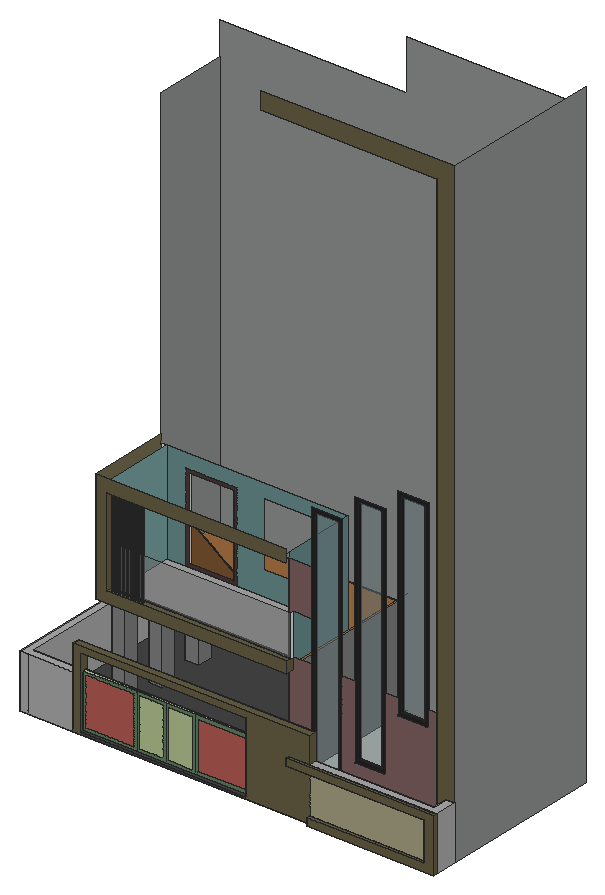
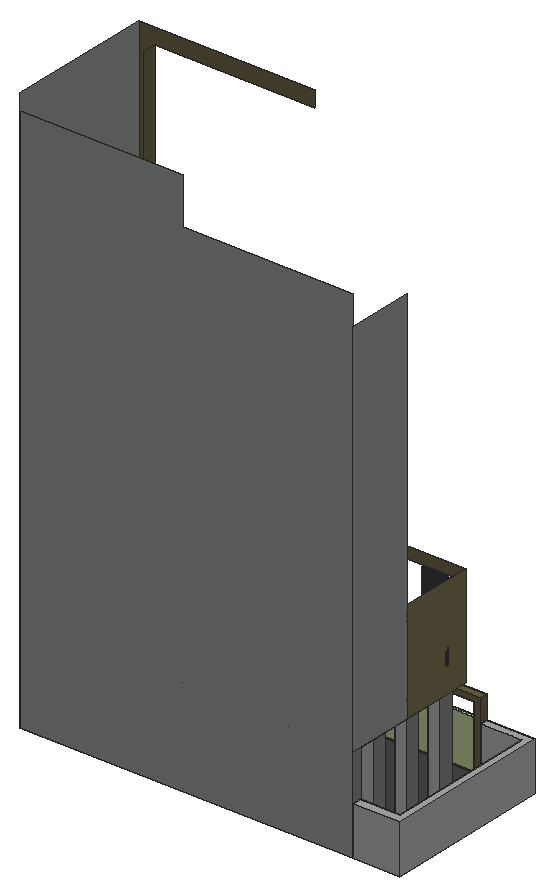
# SketchUp Ruby script. Lengths in inches.
U = 1.inch
M = Sketchup.active_model
def pt(a) = Geom::Point3d.new(a.map { |v| v * U })
def face(e, loops, mat)
  f = e.add_face(loops[0].map { |a| pt(a) })
  loops[1..].each { |l| e.add_face(l.map { |a| pt(a) }).erase! }
  f.material = f.back_material = mat if mat
  f
end
# faces: each face lists its corners as indices into pts; further lists are holes
def faces(e, pts, list, mat = nil) = list.each { |f| face(e, (f[0].is_a?(Array) ? f : [f]).map { |l| l.map { |i| pts[i] } }, mat) }
# xy, xz, yz: faces in a plane at the given z, y or x. An outline is a flat list of corners, or four numbers for a rectangle; further outlines are holes
def ring(l) = l.size == 4 ? [[l[0], l[1]], [l[2], l[1]], [l[2], l[3]], [l[0], l[3]]] : l.each_slice(2).to_a
def flat(e, list, mat, &to3) = list.each { |f| face(e, (f[0].is_a?(Array) ? f : [f]).map { |l| ring(l).map { |u, v| to3.(u, v) } }, mat) }
def xy(e, z, list, mat = nil) = flat(e, list, mat) { |x, y| [x, y, z] }
def xz(e, y, list, mat = nil) = flat(e, list, mat) { |x, z| [x, y, z] }
def yz(e, x, list, mat = nil) = flat(e, list, mat) { |y, z| [x, y, z] }
def lines(e, pts, list) = list.each { |a, b| e.add_line(pt(pts[a]), pt(pts[b])) }
# prism: a flat outline (further loops are holes) pulled along v
def prism(e, loops, v, mat = nil)
  f = face(e, loops, mat); d = Geom::Vector3d.new(v.map { |x| x * U })
  f.pushpull(f.normal.samedirection?(d) ? d.length : -d.length)
end
def box(e, o, s, mat = nil) = prism(e, [[o, [o[0] + s[0], o[1], o[2]], [o[0] + s[0], o[1] + s[1], o[2]], [o[0], o[1] + s[1], o[2]]]], [0, 0, s[2]], mat)
def at(x, y, z, deg = 0) = Geom::Transformation.translation(pt([x, y, z])) * Geom::Transformation.rotation(ORIGIN, Z_AXIS, deg.degrees)
def axes(o, x, y, z) = Geom::Transformation.new([*x, 0, *y, 0, *z, 0, *pt(o).to_a, 1])
def part(name) = M.definitions.add(name)
# library, detail: a bought-in or finely detailed component or shape, given as its bounding box
def library(name, o, s) = part(name).tap { |d| box(d.entities, o, s) }
def detail(e, o, s) = box(e.add_group.entities, o, s)
def put(e, d, t, mat = nil) = e.add_instance(d, t).tap { |i| i.material = mat if mat }
def group(e, t, mat = nil) = e.add_group.tap { |g| g.transformation = t; g.material = mat if mat }.entities
root = M.entities
M.materials.add("[0072_DarkSeaGreen]").color = [96, 127, 96]
M.materials.add("[0089_PaleTurquoise]").color = [103, 140, 140]
M.materials.add("[0089_PaleTurquoise]1").color = [120, 163, 163]
M.materials.add("[0089_PaleTurquoise]2").color = [93, 127, 127]
M.materials.add("[0119_RosyBrown]").color = [127, 96, 96]
M.materials.add("[0119_RosyBrown]1").color = [76, 58, 58]
M.materials.add("[0132_LightGray]").color = [127, 127, 127]
M.materials.add("[0132_LightGray]1").color = [169, 169, 169]
M.materials.add("[0136_Charcoal]").color = [35, 35, 35]
M.materials.add("[Beadboard]").color = [178, 193, 144]
M.materials.add("[Blacktop Old 02]").color = [143, 145, 145]
M.materials.add("[Cladding Siding Tan]").color = [178, 91, 82]
M.materials.add("[Granite Dark Gray]").color = [69, 68, 68]
M.materials.add("[Granite Dark Gray]1").color = [69, 68, 68]
M.materials.add("[Stone Coursed Rough]").color = [165, 160, 130]
M.materials.add("[Stone Vein Gray]").color = [166, 165, 165]
M.materials.add("[Translucent Glass Gray]").color = [130, 130, 130]
M.materials["[Translucent Glass Gray]"].alpha = 0.5
M.materials.add("[Translucent Glass Safety]").color = [119, 137, 142]
M.materials["[Translucent Glass Safety]"].alpha = 0.5
M.materials.add("[Wood Floor]").color = [124, 84, 49]
M.materials.add("[Wood Floor]1").color = [155, 105, 61]
M.materials.add("[Wood Lumber ButtJoined]").color = [102, 94, 69]
M.materials.add("[Wood Lumber ButtJoined]2").color = [117, 108, 80]
xy(root,0,[[0,18,240,894],[240,18,1963.2,198],[240,198,1963.2,894]])
xy(root,0,[[1363.2,0,1963.2,18]],"[Wood Lumber ButtJoined]")
xy(root,12,[[285,32.01,1065,46.01],[249,246,312,318],[249,462,312,534],[249,678,312,750]])
xy(root,12,[[285,18,1065,32.01],[[36,54,1921.2,54,1921.2,126,1879.2,126,1879.2,198,1122,198,1122,846,36,846],[249,462,312,534],[249,246,312,318],[249,678,312,750]]],"[Granite Dark Gray]")
xy(root,12,[[285,46.01,1065,54]],"[Granite Dark Gray]1")
xy(root,30,[[1248,198,1356,208]],"[0136_Charcoal]")
xy(root,36,[[1363.2,0,1915.2,18]],"[Wood Lumber ButtJoined]")
xy(root,220.8,[[1267.2,0,1915.2,18]],"[Wood Lumber ButtJoined]")
xy(root,222,[[1452,198,1560,208]],"[0136_Charcoal]")
xy(root,252,[[0,18,249,18,249,54,36,54,36,846,240,846,240,894,0,894],[1363.2,18,1963.2,18,1963.2,126,1921.2,126,1921.2,54,1363.2,54]],"[0132_LightGray]1")
xy(root,252,[[1267.2,0,1963.2,18]],"[Wood Lumber ButtJoined]")
xy(root,264,[[285,32.01,1065,46.01]],"[Beadboard]")
xy(root,342,[[285,18,1065,54]],"[Wood Lumber ButtJoined]")
xy(root,372,[[249,18,1363.2,54]],"[Wood Lumber ButtJoined]")
xy(root,492,[[[240,198,1122,846],[249,462,312,534],[249,678,312,750],[249,246,312,318]]],"[Wood Floor]1")
xy(root,492,[[240,162,1140.5,198]],"[Wood Lumber ButtJoined]")
xy(root,492.0625,[[1656,198,1764,208]],"[0136_Charcoal]")
xy(root,504,[[270,198,1122,546]],"[Stone Vein Gray]")
xy(root,519.6,[[375.6,546,584.4,551]])
xy(root,546,[[294,189.55,1140.5,198]],"[0089_PaleTurquoise]2")
xy(root,546,[[[294,162,1140.5,189.55],[326.5625,171.77,325.53,171.91,324.5625,172.31,323.73,172.94,323.1,173.77,322.7,174.74,322.5625,175.77,322.7,176.81,323.1,177.77,323.73,178.6,324.5625,179.24,325.53,179.64,326.5625,179.77,327.6,179.64,328.5625,179.24,329.39,178.6,330.03,177.77,330.43,176.81,330.5625,175.77,330.43,174.74,330.03,173.77,329.39,172.94,328.5625,172.31,327.6,171.91],[344.5625,171.77,343.53,171.91,342.5625,172.31,341.73,172.94,341.1,173.77,340.7,174.74,340.5625,175.77,340.7,176.81,341.1,177.77,341.73,178.6,342.5625,179.24,343.53,179.64,344.5625,179.77,345.6,179.64,346.5625,179.24,347.39,178.6,348.03,177.77,348.43,176.81,348.5625,175.77,348.43,174.74,348.03,173.77,347.39,172.94,346.5625,172.31,345.6,171.91],[362.5625,171.77,361.53,171.91,360.5625,172.31,359.73,172.94,359.1,173.77,358.7,174.74,358.5625,175.77,358.7,176.81,359.1,177.77,359.73,178.6,360.5625,179.24,361.53,179.64,362.5625,179.77,363.6,179.64,364.5625,179.24,365.39,178.6,366.03,177.77,366.43,176.81,366.5625,175.77,366.43,174.74,366.03,173.77,365.39,172.94,364.5625,172.31,363.6,171.91],[380.5625,171.77,379.53,171.91,378.5625,172.31,377.73,172.94,377.1,173.77,376.7,174.74,376.5625,175.77,376.7,176.81,377.1,177.77,377.73,178.6,378.5625,179.24,379.53,179.64,380.5625,179.77,381.6,179.64,382.5625,179.24,383.39,178.6,384.03,177.77,384.43,176.81,384.5625,175.77,384.43,174.74,384.03,173.77,383.39,172.94,382.5625,172.31,381.6,171.91],[398.5625,171.77,397.53,171.91,396.5625,172.31,395.73,172.94,395.1,173.77,394.7,174.74,394.5625,175.77,394.7,176.81,395.1,177.77,395.73,178.6,396.5625,179.24,397.53,179.64,398.5625,179.77,399.6,179.64,400.5625,179.24,401.39,178.6,402.03,177.77,402.43,176.81,402.5625,175.77,402.43,174.74,402.03,173.77,401.39,172.94,400.5625,172.31,399.6,171.91],[416.5625,171.77,415.53,171.91,414.5625,172.31,413.73,172.94,413.1,173.77,412.7,174.74,412.5625,175.77,412.7,176.81,413.1,177.77,413.73,178.6,414.5625,179.24,415.53,179.64,416.5625,179.77,417.6,179.64,418.5625,179.24,419.39,178.6,420.03,177.77,420.43,176.81,420.5625,175.77,420.43,174.74,420.03,173.77,419.39,172.94,418.5625,172.31,417.6,171.91],[434.5625,171.77,433.53,171.91,432.5625,172.31,431.73,172.94,431.1,173.77,430.7,174.74,430.5625,175.77,430.7,176.81,431.1,177.77,431.73,178.6,432.5625,179.24,433.53,179.64,434.5625,179.77,435.6,179.64,436.5625,179.24,437.39,178.6,438.03,177.77,438.43,176.81,438.5625,175.77,438.43,174.74,438.03,173.77,437.39,172.94,436.5625,172.31,435.6,171.91],[452.5625,171.77,451.53,171.91,450.5625,172.31,449.73,172.94,449.1,173.77,448.7,174.74,448.5625,175.77,448.7,176.81,449.1,177.77,449.73,178.6,450.5625,179.24,451.53,179.64,452.5625,179.77,453.6,179.64,454.5625,179.24,455.39,178.6,456.03,177.77,456.43,176.81,456.5625,175.77,456.43,174.74,456.03,173.77,455.39,172.94,454.5625,172.31,453.6,171.91],[308.5625,171.77,307.53,171.91,306.5625,172.31,305.73,172.94,305.1,173.77,304.7,174.74,304.5625,175.77,304.7,176.81,305.1,177.77,305.73,178.6,306.5625,179.24,307.53,179.64,308.5625,179.77,309.6,179.64,310.5625,179.24,311.39,178.6,312.03,177.77,312.43,176.81,312.5625,175.77,312.43,174.74,312.03,173.77,311.39,172.94,310.5625,172.31,309.6,171.91]]],"[Wood Lumber ButtJoined]")
xz(root,0,[[1363.2,0,1963.2,0,1963.2,252,1267.2,252,1267.2,220.8,1915.2,220.8,1915.2,36,1363.2,36]],"[Wood Lumber ButtJoined]")
xz(root,18,[[1363.2,0,1363.2,36,1915.2,36,1915.2,220.8,1267.2,220.8,1267.2,252,1963.2,252,1963.2,0]])
xz(root,18,[[0,0,36,252],[36,0,249,252]],"[0132_LightGray]1")
xz(root,18,[[285,0,1065,12]],"[Granite Dark Gray]")
xz(root,18,[[1363.2,36,1915.2,220.8]],"[Stone Coursed Rough]")
xz(root,18,[[249,0,285,0,285,342,1065,342,1065,0,1363.2,0,1363.2,220.8,1267.2,220.8,1267.2,252,1363.2,252,1363.2,372,249,372]],"[Wood Lumber ButtJoined]")
xz(root,32.01,[[[285,12,537,264],[299.4,26.4,522.6,249.6]],[[537,12,675,264],[551.4,26.4,660.6,249.6]],[[675,12,813,264],[689.4,26.4,798.6,249.6]],[[813,12,1065,264],[827.4,26.4,1050.6,249.6]]],"[0072_DarkSeaGreen]")
xz(root,32.01,[[551.4,26.4,660.6,249.6],[689.4,26.4,798.6,249.6]],"[Beadboard]")
xz(root,32.01,[[299.4,26.4,522.6,249.6],[827.4,26.4,1050.6,249.6]],"[Cladding Siding Tan]")
xz(root,46.01,[[285,12,1065,264]],"[Beadboard]")
xz(root,54,[[36,12,249,252],[1363.2,12,1921.2,252]],"[0132_LightGray]1")
xz(root,54,[[249,12,249,372,1363.2,372,1363.2,12,1065,12,1065,342,285,342,285,12]],"[Wood Lumber ButtJoined]")
xz(root,126,[[1921.2,12,1963.2,252]])
xz(root,126,[[1879.2,12,1921.2,12,1921.2,252,1963.2,252,1963.2,2940,1050,2940,1050,2856,1879.2,2856]],"[Wood Lumber ButtJoined]")
xz(root,162,[[240,492,1140.5,492,1140.5,546,294,546,294,960,1135.625,960,1135.625,1020,240,1020]],"[Wood Lumber ButtJoined]")
xz(root,189.55,[[294,546,1140.5,738]],"[Translucent Glass Gray]")
xz(root,198,[[1122,504,1140.5,546]])
xz(root,198,[[270,504,270,960,294,960,294,546,1122,546,1122,504]],"[0089_PaleTurquoise]2")
xz(root,198,[[1122,12,1230,12,1230,549.1875,1140.5,549.1875,1140.5,492,1122,492],[1374,12,1879.2,12,1879.2,549.1875,1782,549.1875,1782,474.0625,1638,474.0625,1638,549.1875,1578,549.1875,1578,204,1434,204,1434,549.1875,1374,549.1875],[1122,546,1140.5,546,1140.5,732,1138.98,732.2,1137.53,732.79,1136.28,733.73,1135.32,734.97,1134.71,736.42,1134.5,737.97,1134.7,739.52,1135.29,740.97,1136.23,742.22,1137.47,743.18,1138.92,743.79,1140.47,744,1142.02,743.8,1143.47,743.21,1144.72,742.27,1230,742.375,1230,958.375,1122,958.375]],"[0119_RosyBrown]")
xz(root,198,[[[1230,12,1374,1212],[1248,30,1356,1194]],[[1434,204,1578,1328.4375],[1452,222,1560,1310.4375]],[[1638,474.0625,1782,1424.375],[1656,492.0625,1764,1406.375]]],"[0136_Charcoal]")
xz(root,208,[[1248,30,1356,1194],[1452,222,1560,1310.4375],[1656,492.0625,1764,1406.375]],"[Translucent Glass Safety]")
xz(root,246,[[249,12,312,492]],"[0132_LightGray]")
xz(root,318,[[249,12,312,492]],"[0132_LightGray]1")
xz(root,462,[[249,12,312,492]],"[0132_LightGray]")
xz(root,534,[[249,12,312,492]],"[0132_LightGray]1")
xz(root,546,[[240,504,270,984]])
xz(root,546,[[[270,504,360,504,360,919.5,600,919.5,600,504,1122,504,1122,984,270,984],[726,619.5,973.25,919.5]]],"[0089_PaleTurquoise]")
xz(root,546,[[[360,504,600,919.5],[375.6,519.6,584.4,903.9]]],"[0119_RosyBrown]1")
xz(root,551,[[584.4,546.38,584.4,551.94,507.28,606.22,503.9375,608.57,379.5,696.14,375.6,692.98]])
xz(root,551,[[375.6,519.6,584.4,519.6,584.4,546.38,375.6,692.98]],"[Wood Floor]")
xz(root,678,[[249,12,312,492]],"[0132_LightGray]")
xz(root,750,[[249,12,312,492]],"[0132_LightGray]1")
xz(root,846,[[240,12,1122,492]],"[0132_LightGray]")
xz(root,846,[[36,12,240,252]],"[0132_LightGray]1")
xz(root,894,[[0,0,240,252]],"[0132_LightGray]1")
xz(root,894,[[240,0,240,2616,1122,2616,1122,2856,1963.2,2856,1963.2,0]],"[Blacktop Old 02]")
yz(root,0,[[18,0,894,252]],"[0132_LightGray]1")
yz(root,36,[[54,12,846,252]],"[0132_LightGray]1")
yz(root,240,[[846,12,894,252]])
yz(root,240,[[846,252,894,492]],"[0132_LightGray]")
yz(root,240,[[546,492,894,2460]],"[Blacktop Old 02]")
yz(root,240,[[162,492,546,1020]],"[Wood Lumber ButtJoined]2")
yz(root,249,[[18,12,54,252]])
yz(root,249,[[246,12,318,492],[462,12,534,492],[678,12,750,492]],"[0132_LightGray]")
yz(root,249,[[18,252,54,372]],"[Wood Lumber ButtJoined]")
yz(root,270,[[198,504,546,504,546,984,204,984,204,960,198,960]],"[0089_PaleTurquoise]1")
yz(root,285,[[32.01,12,46.01,264]])
yz(root,285,[[18,12,32.01,12,32.01,264,46.01,264,46.01,12,54,12,54,342,18,342]],"[Wood Lumber ButtJoined]")
yz(root,294,[[[162,546,198,960],[189.51,732,187.96,732.21,186.52,732.82,185.28,733.78,184.33,735.03,183.74,736.48,183.55,738.03,183.76,739.58,184.37,741.03,185.33,742.27,186.57,743.21,188.02,743.8,189.58,744,191.13,743.79,192.57,743.18,193.8125,742.22,194.76,740.97,195.35,739.52,195.55,737.97,195.33,736.42,194.72,734.97,193.76,733.73,192.52,732.79,191.07,732.2,189.55,732]]],"[Wood Lumber ButtJoined]")
yz(root,312,[[246,12,318,492],[462,12,534,492],[678,12,750,492]],"[0132_LightGray]")
yz(root,375.6,[[546,519.6,551,903.9]])
yz(root,584.4,[[546,519.6,551,903.9]])
yz(root,1065,[[32.01,12,46.01,264]])
yz(root,1065,[[18,12,18,342,54,342,54,12,46.01,12,46.01,264,32.01,264,32.01,12]],"[Wood Lumber ButtJoined]")
yz(root,1122,[[198,504,198,960,204,960,204,984,546,984,546,504]],"[0089_PaleTurquoise]")
yz(root,1122,[[198,12,846,492]],"[0132_LightGray]")
yz(root,1140.5,[[189.55,546,198,738]])
yz(root,1140.5,[[162,492,198,546]],"[Wood Lumber ButtJoined]")
yz(root,1248,[[198,30,208,1194]],"[0136_Charcoal]")
yz(root,1267.2,[[0,220.8,18,252]],"[Wood Lumber ButtJoined]")
yz(root,1356,[[198,30,208,1194]],"[0136_Charcoal]")
yz(root,1363.2,[[0,0,18,36],[18,252,54,372]],"[Wood Lumber ButtJoined]")
yz(root,1452,[[198,222,208,1310.4375]],"[0136_Charcoal]")
yz(root,1560,[[198,222,208,1310.4375]],"[0136_Charcoal]")
yz(root,1656,[[198,492.0625,208,1406.375]],"[0136_Charcoal]")
yz(root,1764,[[198,492.0625,208,1406.375]],"[0136_Charcoal]")
yz(root,1879.2,[[126,12,198,2856]],"[Wood Lumber ButtJoined]")
yz(root,1915.2,[[0,36,18,220.8]],"[Wood Lumber ButtJoined]")
yz(root,1921.2,[[54,12,126,252]],"[0132_LightGray]1")
yz(root,1963.2,[[18,0,126,252]],"[0132_LightGray]1")
yz(root,1963.2,[[126,0,894,2940]],"[Blacktop Old 02]")
yz(root,1963.2,[[0,0,18,252]],"[Wood Lumber ButtJoined]")
p = [[307.53,171.91,546],[308.5625,171.77,546],[308.5625,171.77,960],[307.53,171.91,960],[309.6,171.91,546],[309.6,171.91,960],
  [325.53,171.91,546],[326.5625,171.77,546],[326.5625,171.77,960],[325.53,171.91,960],[327.6,171.91,546],[327.6,171.91,960],
  [343.53,171.91,546],[344.5625,171.77,546],[344.5625,171.77,960],[343.53,171.91,960],[345.6,171.91,546],[345.6,171.91,960],
  [361.53,171.91,546],[362.5625,171.77,546],[362.5625,171.77,960],[361.53,171.91,960],[363.6,171.91,546],[363.6,171.91,960],
  [379.53,171.91,546],[380.5625,171.77,546],[380.5625,171.77,960],[379.53,171.91,960],[381.6,171.91,546],[381.6,171.91,960],
  [397.53,171.91,546],[398.5625,171.77,546],[398.5625,171.77,960],[397.53,171.91,960],[399.6,171.91,546],[399.6,171.91,960],
  [415.53,171.91,546],[416.5625,171.77,546],[416.5625,171.77,960],[415.53,171.91,960],[417.6,171.91,546],[417.6,171.91,960],
  [433.53,171.91,546],[434.5625,171.77,546],[434.5625,171.77,960],[433.53,171.91,960],[435.6,171.91,546],[435.6,171.91,960],
  [451.53,171.91,546],[452.5625,171.77,546],[452.5625,171.77,960],[451.53,171.91,960],[453.6,171.91,546],[453.6,171.91,960],
  [306.5625,172.31,546],[306.5625,172.31,960],[310.5625,172.31,546],[310.5625,172.31,960],[324.5625,172.31,546],[324.5625,172.31,960],
  [328.5625,172.31,546],[328.5625,172.31,960],[342.5625,172.31,546],[342.5625,172.31,960],[346.5625,172.31,546],[346.5625,172.31,960],
  [360.5625,172.31,546],[360.5625,172.31,960],[364.5625,172.31,546],[364.5625,172.31,960],[378.5625,172.31,546],[378.5625,172.31,960],
  [382.5625,172.31,546],[382.5625,172.31,960],[396.5625,172.31,546],[396.5625,172.31,960],[400.5625,172.31,546],[400.5625,172.31,960],
  [414.5625,172.31,546],[414.5625,172.31,960],[418.5625,172.31,546],[418.5625,172.31,960],[432.5625,172.31,546],[432.5625,172.31,960],
  [436.5625,172.31,546],[436.5625,172.31,960],[450.5625,172.31,546],[450.5625,172.31,960],[454.5625,172.31,546],[454.5625,172.31,960],
  [305.73,172.94,546],[305.73,172.94,960],[311.39,172.94,546],[311.39,172.94,960],[323.73,172.94,546],[323.73,172.94,960],
  [329.39,172.94,546],[329.39,172.94,960],[341.73,172.94,546],[341.73,172.94,960],[347.39,172.94,546],[347.39,172.94,960],
  [359.73,172.94,546],[359.73,172.94,960],[365.39,172.94,546],[365.39,172.94,960],[377.73,172.94,546],[377.73,172.94,960],
  [383.39,172.94,546],[383.39,172.94,960],[395.73,172.94,546],[395.73,172.94,960],[401.39,172.94,546],[401.39,172.94,960],
  [413.73,172.94,546],[413.73,172.94,960],[419.39,172.94,546],[419.39,172.94,960],[431.73,172.94,546],[431.73,172.94,960],
  [437.39,172.94,546],[437.39,172.94,960],[449.73,172.94,546],[449.73,172.94,960],[455.39,172.94,546],[455.39,172.94,960],
  [305.1,173.77,546],[305.1,173.77,960],[312.03,173.77,546],[312.03,173.77,960],[323.1,173.77,546],[323.1,173.77,960],
  [330.03,173.77,546],[330.03,173.77,960],[341.1,173.77,546],[341.1,173.77,960],[348.03,173.77,546],[348.03,173.77,960],
  [359.1,173.77,546],[359.1,173.77,960],[366.03,173.77,546],[366.03,173.77,960],[377.1,173.77,546],[377.1,173.77,960],
  [384.03,173.77,546],[384.03,173.77,960],[395.1,173.77,546],[395.1,173.77,960],[402.03,173.77,546],[402.03,173.77,960],
  [413.1,173.77,546],[413.1,173.77,960],[420.03,173.77,546],[420.03,173.77,960],[431.1,173.77,546],[431.1,173.77,960],
  [438.03,173.77,546],[438.03,173.77,960],[449.1,173.77,546],[449.1,173.77,960],[456.03,173.77,546],[456.03,173.77,960],
  [304.7,174.74,546],[304.7,174.74,960],[312.43,174.74,546],[312.43,174.74,960],[322.7,174.74,546],[322.7,174.74,960],
  [330.43,174.74,546],[330.43,174.74,960],[340.7,174.74,546],[340.7,174.74,960],[348.43,174.74,546],[348.43,174.74,960],
  [358.7,174.74,546],[358.7,174.74,960],[366.43,174.74,546],[366.43,174.74,960],[376.7,174.74,546],[376.7,174.74,960],
  [384.43,174.74,546],[384.43,174.74,960],[394.7,174.74,546],[394.7,174.74,960],[402.43,174.74,546],[402.43,174.74,960],
  [412.7,174.74,546],[412.7,174.74,960],[420.43,174.74,546],[420.43,174.74,960],[430.7,174.74,546],[430.7,174.74,960],
  [438.43,174.74,546],[438.43,174.74,960],[448.7,174.74,546],[448.7,174.74,960],[456.43,174.74,546],[456.43,174.74,960],
  [304.5625,175.77,546],[304.5625,175.77,960],[312.5625,175.77,546],[312.5625,175.77,960],[322.5625,175.77,546],[322.5625,175.77,960],
  [330.5625,175.77,546],[330.5625,175.77,960],[340.5625,175.77,546],[340.5625,175.77,960],[348.5625,175.77,546],[348.5625,175.77,960],
  [358.5625,175.77,546],[358.5625,175.77,960],[366.5625,175.77,546],[366.5625,175.77,960],[376.5625,175.77,546],[376.5625,175.77,960],
  [384.5625,175.77,546],[384.5625,175.77,960],[394.5625,175.77,546],[394.5625,175.77,960],[402.5625,175.77,546],[402.5625,175.77,960],
  [412.5625,175.77,546],[412.5625,175.77,960],[420.5625,175.77,546],[420.5625,175.77,960],[430.5625,175.77,546],[430.5625,175.77,960],
  [438.5625,175.77,546],[438.5625,175.77,960],[448.5625,175.77,546],[448.5625,175.77,960],[456.5625,175.77,546],[456.5625,175.77,960],
  [304.7,176.81,546],[304.7,176.81,960],[312.43,176.81,546],[312.43,176.81,960],[322.7,176.81,546],[322.7,176.81,960],
  [330.43,176.81,546],[330.43,176.81,960],[340.7,176.81,546],[340.7,176.81,960],[348.43,176.81,546],[348.43,176.81,960],
  [358.7,176.81,546],[358.7,176.81,960],[366.43,176.81,546],[366.43,176.81,960],[376.7,176.81,546],[376.7,176.81,960],
  [384.43,176.81,546],[384.43,176.81,960],[394.7,176.81,546],[394.7,176.81,960],[402.43,176.81,546],[402.43,176.81,960],
  [412.7,176.81,546],[412.7,176.81,960],[420.43,176.81,546],[420.43,176.81,960],[430.7,176.81,546],[430.7,176.81,960],
  [438.43,176.81,546],[438.43,176.81,960],[448.7,176.81,546],[448.7,176.81,960],[456.43,176.81,546],[456.43,176.81,960],
  [305.1,177.77,546],[305.1,177.77,960],[312.03,177.77,546],[312.03,177.77,960],[323.1,177.77,546],[323.1,177.77,960],
  [330.03,177.77,546],[330.03,177.77,960],[341.1,177.77,546],[341.1,177.77,960],[348.03,177.77,546],[348.03,177.77,960],
  [359.1,177.77,546],[359.1,177.77,960],[366.03,177.77,546],[366.03,177.77,960],[377.1,177.77,546],[377.1,177.77,960],
  [384.03,177.77,546],[384.03,177.77,960],[395.1,177.77,546],[395.1,177.77,960],[402.03,177.77,546],[402.03,177.77,960],
  [413.1,177.77,546],[413.1,177.77,960],[420.03,177.77,546],[420.03,177.77,960],[431.1,177.77,546],[431.1,177.77,960],
  [438.03,177.77,546],[438.03,177.77,960],[449.1,177.77,546],[449.1,177.77,960],[456.03,177.77,546],[456.03,177.77,960],
  [305.73,178.6,546],[305.73,178.6,960],[311.39,178.6,546],[311.39,178.6,960],[323.73,178.6,546],[323.73,178.6,960],
  [329.39,178.6,546],[329.39,178.6,960],[341.73,178.6,546],[341.73,178.6,960],[347.39,178.6,546],[347.39,178.6,960],
  [359.73,178.6,546],[359.73,178.6,960],[365.39,178.6,546],[365.39,178.6,960],[377.73,178.6,546],[377.73,178.6,960],
  [383.39,178.6,546],[383.39,178.6,960],[395.73,178.6,546],[395.73,178.6,960],[401.39,178.6,546],[401.39,178.6,960],
  [413.73,178.6,546],[413.73,178.6,960],[419.39,178.6,546],[419.39,178.6,960],[431.73,178.6,546],[431.73,178.6,960],
  [437.39,178.6,546],[437.39,178.6,960],[449.73,178.6,546],[449.73,178.6,960],[455.39,178.6,546],[455.39,178.6,960],
  [306.5625,179.24,546],[306.5625,179.24,960],[310.5625,179.24,546],[310.5625,179.24,960],[324.5625,179.24,546],[324.5625,179.24,960],
  [328.5625,179.24,546],[328.5625,179.24,960],[342.5625,179.24,546],[342.5625,179.24,960],[346.5625,179.24,546],[346.5625,179.24,960],
  [360.5625,179.24,546],[360.5625,179.24,960],[364.5625,179.24,546],[364.5625,179.24,960],[378.5625,179.24,546],[378.5625,179.24,960],
  [382.5625,179.24,546],[382.5625,179.24,960],[396.5625,179.24,546],[396.5625,179.24,960],[400.5625,179.24,546],[400.5625,179.24,960],
  [414.5625,179.24,546],[414.5625,179.24,960],[418.5625,179.24,546],[418.5625,179.24,960],[432.5625,179.24,546],[432.5625,179.24,960],
  [436.5625,179.24,546],[436.5625,179.24,960],[450.5625,179.24,546],[450.5625,179.24,960],[454.5625,179.24,546],[454.5625,179.24,960],
  [307.53,179.64,546],[307.53,179.64,960],[309.6,179.64,546],[309.6,179.64,960],[325.53,179.64,546],[325.53,179.64,960],
  [327.6,179.64,546],[327.6,179.64,960],[343.53,179.64,546],[343.53,179.64,960],[345.6,179.64,546],[345.6,179.64,960],
  [361.53,179.64,546],[361.53,179.64,960],[363.6,179.64,546],[363.6,179.64,960],[379.53,179.64,546],[379.53,179.64,960],
  [381.6,179.64,546],[381.6,179.64,960],[397.53,179.64,546],[397.53,179.64,960],[399.6,179.64,546],[399.6,179.64,960],
  [415.53,179.64,546],[415.53,179.64,960],[417.6,179.64,546],[417.6,179.64,960],[433.53,179.64,546],[433.53,179.64,960],
  [435.6,179.64,546],[435.6,179.64,960],[451.53,179.64,546],[451.53,179.64,960],[453.6,179.64,546],[453.6,179.64,960],
  [308.5625,179.77,546],[308.5625,179.77,960],[326.5625,179.77,546],[326.5625,179.77,960],[344.5625,179.77,546],[344.5625,179.77,960],
  [362.5625,179.77,546],[362.5625,179.77,960],[380.5625,179.77,546],[380.5625,179.77,960],[398.5625,179.77,546],[398.5625,179.77,960],
  [416.5625,179.77,546],[416.5625,179.77,960],[434.5625,179.77,546],[434.5625,179.77,960],[452.5625,179.77,546],[452.5625,179.77,960],
  [1122,846,12],[1122,894,12],[576,846,492],[576,894,492],[1122,546,504],[1122,894,504],
  [270,198,504],[240,198,504],[1879.2,198,12],[1879.2,198,0],[36,54,12],[36,18,12],
  [1363.2,54,12],[1363.2,18,12]]
faces(root,p,[[0,1,2,3],[1,4,5,2],[6,7,8,9],[7,10,11,8],[12,13,14,15],[13,16,17,14],[18,19,20,21],[19,22,23,20],
  [24,25,26,27],[25,28,29,26],[30,31,32,33],[31,34,35,32],[36,37,38,39],[37,40,41,38],[42,43,44,45],[43,46,47,44],
  [48,49,50,51],[49,52,53,50],[54,0,3,55],[4,56,57,5],[58,6,9,59],[10,60,61,11],[62,12,15,63],[16,64,65,17],
  [66,18,21,67],[22,68,69,23],[70,24,27,71],[28,72,73,29],[74,30,33,75],[34,76,77,35],[78,36,39,79],[40,80,81,41],
  [82,42,45,83],[46,84,85,47],[86,48,51,87],[52,88,89,53],[90,54,55,91],[56,92,93,57],[94,58,59,95],[60,96,97,61],
  [98,62,63,99],[64,100,101,65],[102,66,67,103],[68,104,105,69],[106,70,71,107],[72,108,109,73],[110,74,75,111],[76,112,113,77],
  [114,78,79,115],[80,116,117,81],[118,82,83,119],[84,120,121,85],[122,86,87,123],[88,124,125,89],[126,90,91,127],[92,128,129,93],
  [130,94,95,131],[96,132,133,97],[134,98,99,135],[100,136,137,101],[138,102,103,139],[104,140,141,105],[142,106,107,143],[108,144,145,109],
  [146,110,111,147],[112,148,149,113],[150,114,115,151],[116,152,153,117],[154,118,119,155],[120,156,157,121],[158,122,123,159],[124,160,161,125],
  [162,126,127,163],[128,164,165,129],[166,130,131,167],[132,168,169,133],[170,134,135,171],[136,172,173,137],[174,138,139,175],[140,176,177,141],
  [178,142,143,179],[144,180,181,145],[182,146,147,183],[148,184,185,149],[186,150,151,187],[152,188,189,153],[190,154,155,191],[156,192,193,157],
  [194,158,159,195],[160,196,197,161],[198,162,163,199],[164,200,201,165],[202,166,167,203],[168,204,205,169],[206,170,171,207],[172,208,209,173],
  [210,174,175,211],[176,212,213,177],[214,178,179,215],[180,216,217,181],[218,182,183,219],[184,220,221,185],[222,186,187,223],[188,224,225,189],
  [226,190,191,227],[192,228,229,193],[230,194,195,231],[196,232,233,197],[234,198,199,235],[200,236,237,201],[238,202,203,239],[204,240,241,205],
  [242,206,207,243],[208,244,245,209],[246,210,211,247],[212,248,249,213],[250,214,215,251],[216,252,253,217],[254,218,219,255],[220,256,257,221],
  [258,222,223,259],[224,260,261,225],[262,226,227,263],[228,264,265,229],[266,230,231,267],[232,268,269,233],[270,234,235,271],[236,272,273,237],
  [274,238,239,275],[240,276,277,241],[278,242,243,279],[244,280,281,245],[282,246,247,283],[248,284,285,249],[286,250,251,287],[252,288,289,253],
  [290,254,255,291],[256,292,293,257],[294,258,259,295],[260,296,297,261],[298,262,263,299],[264,300,301,265],[302,266,267,303],[268,304,305,269],
  [306,270,271,307],[272,308,309,273],[310,274,275,311],[276,312,313,277],[314,278,279,315],[280,316,317,281],[318,282,283,319],[284,320,321,285],
  [322,286,287,323],[288,324,325,289],[326,290,291,327],[292,328,329,293],[330,294,295,331],[296,332,333,297],[334,298,299,335],[300,336,337,301],
  [338,302,303,339],[304,340,341,305],[342,306,307,343],[308,344,345,309],[346,310,311,347],[312,348,349,313],[350,314,315,351],[316,352,353,317],
  [354,318,319,355],[320,356,357,321],[358,322,323,359],[324,360,361,325],[362,326,327,363],[328,364,365,329],[366,330,331,367],[332,368,369,333],
  [370,334,335,371],[336,372,373,337],[374,338,339,375],[340,376,377,341],[378,342,343,379],[344,380,381,345],[382,346,347,383],[348,384,385,349],
  [386,350,351,387],[352,388,389,353],[390,354,355,391],[356,392,393,357],[394,358,359,395],[360,396,397,361],[398,362,363,399],[364,400,401,365],
  [402,366,367,403],[368,404,405,369],[406,370,371,407],[372,408,409,373],[410,374,375,411],[376,412,413,377],[414,378,379,415],[380,414,415,381],
  [416,382,383,417],[384,416,417,385],[418,386,387,419],[388,418,419,389],[420,390,391,421],[392,420,421,393],[422,394,395,423],[396,422,423,397],
  [424,398,399,425],[400,424,425,401],[426,402,403,427],[404,426,427,405],[428,406,407,429],[408,428,429,409],[430,410,411,431],[412,430,431,413]],"[0119_RosyBrown]")
lines(root,p,[[432,433],[434,435],[436,437],[438,439],[440,441],[442,443],[444,445]])
